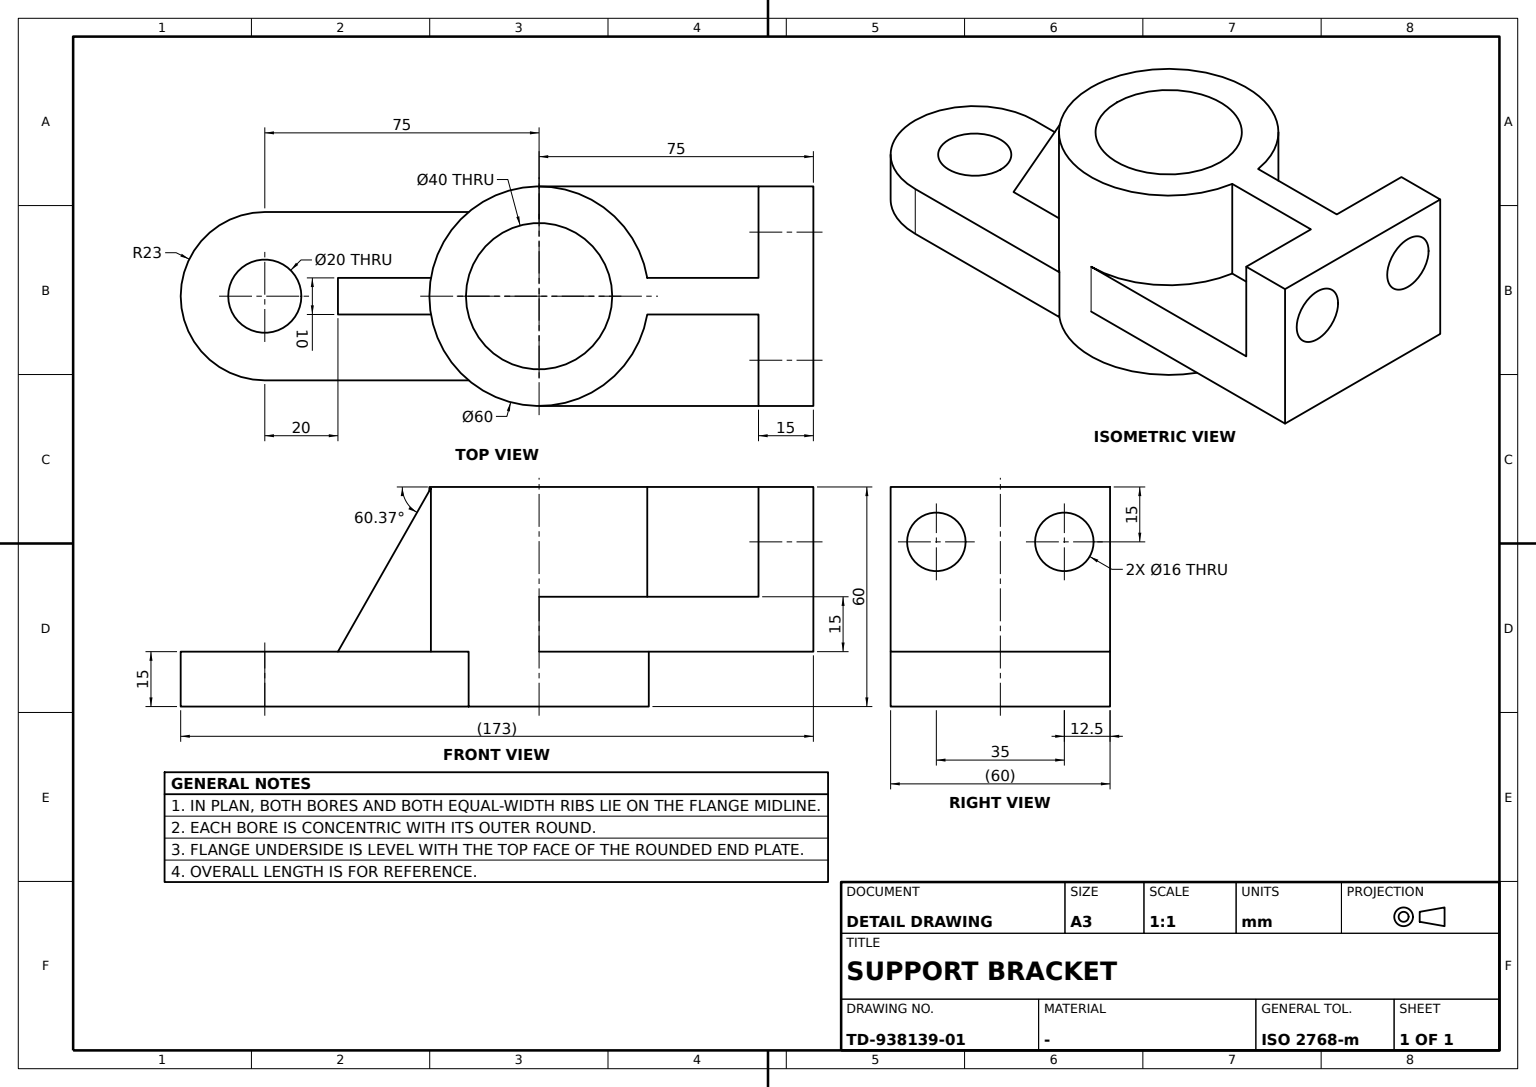
ISO-10303-21;
HEADER;
FILE_DESCRIPTION((''),'2;1');
FILE_NAME('','',(''),(''),'','','');
FILE_SCHEMA(('AUTOMOTIVE_DESIGN'));
ENDSEC;
DATA;
#1=APPLICATION_CONTEXT('');
#2=PRODUCT_CONTEXT('',#1,'mechanical');
#3=PRODUCT('','','',(#2));
#4=PRODUCT_DEFINITION_FORMATION('','',#3);
#5=PRODUCT_DEFINITION_CONTEXT('',#1,'design');
#6=PRODUCT_DEFINITION('','',#4,#5);
#7=PRODUCT_DEFINITION_SHAPE('','',#6);
#8=(LENGTH_UNIT()NAMED_UNIT(*)SI_UNIT(.MILLI.,.METRE.));
#9=(NAMED_UNIT(*)PLANE_ANGLE_UNIT()SI_UNIT($,.RADIAN.));
#10=(NAMED_UNIT(*)SI_UNIT($,.STERADIAN.)SOLID_ANGLE_UNIT());
#11=UNCERTAINTY_MEASURE_WITH_UNIT(LENGTH_MEASURE(1.E-05),#8,'distance_accuracy_value','');
#12=(GEOMETRIC_REPRESENTATION_CONTEXT(3)GLOBAL_UNCERTAINTY_ASSIGNED_CONTEXT((#11))GLOBAL_UNIT_ASSIGNED_CONTEXT((#8,#9,#10))REPRESENTATION_CONTEXT('',''));
#13=CARTESIAN_POINT('',(55.,-5.,15.));
#14=VERTEX_POINT('',#13);
#15=CARTESIAN_POINT('',(55.,5.,15.));
#16=VERTEX_POINT('',#15);
#17=CARTESIAN_POINT('',(55.,0.,15.));
#18=DIRECTION('',(0.,1.,0.));
#19=VECTOR('',#18,1000.);
#20=LINE('',#17,#19);
#21=EDGE_CURVE('',#14,#16,#20,.T.);
#22=ORIENTED_EDGE('',*,*,#21,.T.);
#23=CARTESIAN_POINT('',(29.580399,5.,59.691972));
#24=VERTEX_POINT('',#23);
#25=CARTESIAN_POINT('',(42.290199,5.,37.345986));
#26=DIRECTION('',(0.494398032,0.,-0.869235633));
#27=VECTOR('',#26,1000.);
#28=LINE('',#25,#27);
#29=EDGE_CURVE('',#24,#16,#28,.T.);
#30=ORIENTED_EDGE('',*,*,#29,.F.);
#31=CARTESIAN_POINT('',(30.,0.,58.954242));
#32=VERTEX_POINT('',#31);
#33=CARTESIAN_POINT('',(30.,1.019035,58.954242));
#34=CARTESIAN_POINT('',(29.956732,2.038069,59.030315));
#35=CARTESIAN_POINT('',(29.870188,3.046505,59.182474));
#36=CARTESIAN_POINT('',(29.743385,4.035763,59.405415));
#37=B_SPLINE_CURVE_WITH_KNOTS('',5,(#31,#33,#34,#35,#36,#23),.UNSPECIFIED.,.F.,.F.,(6,6),(0.,7.205662734),.UNSPECIFIED.);
#38=EDGE_CURVE('',#32,#24,#37,.T.);
#39=ORIENTED_EDGE('',*,*,#38,.F.);
#40=CARTESIAN_POINT('',(29.580399,-5.,59.691972));
#41=VERTEX_POINT('',#40);
#42=CARTESIAN_POINT('',(30.,-1.019035,58.954242));
#43=CARTESIAN_POINT('',(29.956732,-2.038069,59.030315));
#44=CARTESIAN_POINT('',(29.870188,-3.046505,59.182474));
#45=CARTESIAN_POINT('',(29.743385,-4.035763,59.405415));
#46=B_SPLINE_CURVE_WITH_KNOTS('',5,(#31,#42,#43,#44,#45,#40),.UNSPECIFIED.,.F.,.F.,(6,6),(0.,7.205662735),.UNSPECIFIED.);
#47=EDGE_CURVE('',#32,#41,#46,.T.);
#48=ORIENTED_EDGE('',*,*,#47,.T.);
#49=CARTESIAN_POINT('',(42.290199,-5.,37.345986));
#50=LINE('',#49,#27);
#51=EDGE_CURVE('',#41,#14,#50,.T.);
#52=ORIENTED_EDGE('',*,*,#51,.T.);
#53=EDGE_LOOP('',(#22,#30,#39,#48,#52));
#54=FACE_OUTER_BOUND('',#53,.T.);
#55=CARTESIAN_POINT('',(29.60858,0.,59.642426));
#56=DIRECTION('',(-0.869235633,0.,-0.494398032));
#57=DIRECTION('',(-0.494398032,0.,0.869235633));
#58=AXIS2_PLACEMENT_3D('',#55,#56,#57);
#59=PLANE('',#58);
#60=ADVANCED_FACE('',(#54),#59,.F.);
#61=CARTESIAN_POINT('',(75.,-23.,0.));
#62=VERTEX_POINT('',#61);
#63=CARTESIAN_POINT('',(19.26136,-23.,0.));
#64=VERTEX_POINT('',#63);
#65=CARTESIAN_POINT('',(47.13068,-23.,0.));
#66=DIRECTION('',(-1.,0.,0.));
#67=VECTOR('',#66,1000.);
#68=LINE('',#65,#67);
#69=EDGE_CURVE('',#62,#64,#68,.T.);
#70=ORIENTED_EDGE('',*,*,#69,.T.);
#71=CARTESIAN_POINT('',(-30.,0.,0.));
#72=VERTEX_POINT('',#71);
#73=CARTESIAN_POINT('',(0.,0.,0.));
#74=DIRECTION('',(0.,0.,1.));
#75=DIRECTION('',(1.,0.,0.));
#76=AXIS2_PLACEMENT_3D('',#73,#74,#75);
#77=CIRCLE('',#76,30.);
#78=EDGE_CURVE('',#72,#64,#77,.T.);
#79=ORIENTED_EDGE('',*,*,#78,.F.);
#80=CARTESIAN_POINT('',(19.26136,23.,0.));
#81=VERTEX_POINT('',#80);
#82=EDGE_CURVE('',#81,#72,#77,.T.);
#83=ORIENTED_EDGE('',*,*,#82,.F.);
#84=CARTESIAN_POINT('',(75.,23.,0.));
#85=VERTEX_POINT('',#84);
#86=CARTESIAN_POINT('',(47.13068,23.,0.));
#87=VECTOR('',#75,1000.);
#88=LINE('',#86,#87);
#89=EDGE_CURVE('',#81,#85,#88,.T.);
#90=ORIENTED_EDGE('',*,*,#89,.T.);
#91=CARTESIAN_POINT('',(98.,0.,0.));
#92=VERTEX_POINT('',#91);
#93=CARTESIAN_POINT('',(75.,0.,0.));
#94=DIRECTION('',(0.,0.,-1.));
#95=AXIS2_PLACEMENT_3D('',#93,#94,#75);
#96=CIRCLE('',#95,23.);
#97=EDGE_CURVE('',#85,#92,#96,.T.);
#98=ORIENTED_EDGE('',*,*,#97,.T.);
#99=EDGE_CURVE('',#92,#62,#96,.T.);
#100=ORIENTED_EDGE('',*,*,#99,.T.);
#101=EDGE_LOOP('',(#70,#79,#83,#90,#98,#100));
#102=FACE_OUTER_BOUND('',#101,.T.);
#103=CARTESIAN_POINT('',(20.,0.,0.));
#104=VERTEX_POINT('',#103);
#105=CARTESIAN_POINT('',(-20.,0.,0.));
#106=VERTEX_POINT('',#105);
#107=CIRCLE('',#76,20.);
#108=EDGE_CURVE('',#104,#106,#107,.T.);
#109=ORIENTED_EDGE('',*,*,#108,.T.);
#110=EDGE_CURVE('',#106,#104,#107,.T.);
#111=ORIENTED_EDGE('',*,*,#110,.T.);
#112=EDGE_LOOP('',(#109,#111));
#113=FACE_BOUND('',#112,.T.);
#114=CARTESIAN_POINT('',(85.,0.,0.));
#115=VERTEX_POINT('',#114);
#116=CARTESIAN_POINT('',(65.,0.,0.));
#117=VERTEX_POINT('',#116);
#118=AXIS2_PLACEMENT_3D('',#93,#74,#75);
#119=CIRCLE('',#118,10.);
#120=EDGE_CURVE('',#115,#117,#119,.T.);
#121=ORIENTED_EDGE('',*,*,#120,.T.);
#122=EDGE_CURVE('',#117,#115,#119,.T.);
#123=ORIENTED_EDGE('',*,*,#122,.T.);
#124=EDGE_LOOP('',(#121,#123));
#125=FACE_BOUND('',#124,.T.);
#126=PLANE('',#76);
#127=ADVANCED_FACE('',(#102,#113,#125),#126,.F.);
#128=CARTESIAN_POINT('',(-75.,-30.,60.));
#129=VERTEX_POINT('',#128);
#130=CARTESIAN_POINT('',(-75.,30.,60.));
#131=VERTEX_POINT('',#130);
#132=CARTESIAN_POINT('',(-75.,0.,60.));
#133=LINE('',#132,#19);
#134=EDGE_CURVE('',#129,#131,#133,.T.);
#135=ORIENTED_EDGE('',*,*,#134,.F.);
#136=CARTESIAN_POINT('',(-60.,-30.,60.));
#137=VERTEX_POINT('',#136);
#138=CARTESIAN_POINT('',(-67.5,-30.,60.));
#139=LINE('',#138,#87);
#140=EDGE_CURVE('',#129,#137,#139,.T.);
#141=ORIENTED_EDGE('',*,*,#140,.T.);
#142=CARTESIAN_POINT('',(-60.,-5.,60.));
#143=VERTEX_POINT('',#142);
#144=CARTESIAN_POINT('',(-60.,-17.5,60.));
#145=LINE('',#144,#19);
#146=EDGE_CURVE('',#137,#143,#145,.T.);
#147=ORIENTED_EDGE('',*,*,#146,.T.);
#148=CARTESIAN_POINT('',(-60.,5.,60.));
#149=VERTEX_POINT('',#148);
#150=CARTESIAN_POINT('',(-60.,0.,60.));
#151=LINE('',#150,#19);
#152=EDGE_CURVE('',#143,#149,#151,.T.);
#153=ORIENTED_EDGE('',*,*,#152,.T.);
#154=CARTESIAN_POINT('',(-60.,30.,60.));
#155=VERTEX_POINT('',#154);
#156=CARTESIAN_POINT('',(-60.,17.5,60.));
#157=LINE('',#156,#19);
#158=EDGE_CURVE('',#149,#155,#157,.T.);
#159=ORIENTED_EDGE('',*,*,#158,.T.);
#160=CARTESIAN_POINT('',(-67.5,30.,60.));
#161=LINE('',#160,#87);
#162=EDGE_CURVE('',#131,#155,#161,.T.);
#163=ORIENTED_EDGE('',*,*,#162,.F.);
#164=EDGE_LOOP('',(#135,#141,#147,#153,#159,#163));
#165=FACE_OUTER_BOUND('',#164,.T.);
#166=CARTESIAN_POINT('',(0.,0.,60.));
#167=AXIS2_PLACEMENT_3D('',#166,#74,#75);
#168=PLANE('',#167);
#169=ADVANCED_FACE('',(#165),#168,.T.);
#170=CARTESIAN_POINT('',(-75.,9.5,45.));
#171=VERTEX_POINT('',#170);
#172=CARTESIAN_POINT('',(-60.,9.5,45.));
#173=VERTEX_POINT('',#172);
#174=CARTESIAN_POINT('',(-67.5,9.5,45.));
#175=LINE('',#174,#87);
#176=EDGE_CURVE('',#171,#173,#175,.T.);
#177=ORIENTED_EDGE('',*,*,#176,.F.);
#178=CARTESIAN_POINT('',(-75.,25.5,45.));
#179=VERTEX_POINT('',#178);
#180=CARTESIAN_POINT('',(-75.,17.5,45.));
#181=DIRECTION('',(0.,-1.,0.));
#182=AXIS2_PLACEMENT_3D('',#180,#66,#181);
#183=CIRCLE('',#182,8.);
#184=EDGE_CURVE('',#171,#179,#183,.T.);
#185=ORIENTED_EDGE('',*,*,#184,.T.);
#186=CARTESIAN_POINT('',(-60.,25.5,45.));
#187=VERTEX_POINT('',#186);
#188=CARTESIAN_POINT('',(-67.5,25.5,45.));
#189=LINE('',#188,#87);
#190=EDGE_CURVE('',#179,#187,#189,.T.);
#191=ORIENTED_EDGE('',*,*,#190,.T.);
#192=CARTESIAN_POINT('',(-60.,17.5,45.));
#193=AXIS2_PLACEMENT_3D('',#192,#66,#181);
#194=CIRCLE('',#193,8.);
#195=EDGE_CURVE('',#173,#187,#194,.T.);
#196=ORIENTED_EDGE('',*,*,#195,.F.);
#197=EDGE_LOOP('',(#177,#185,#191,#196));
#198=FACE_OUTER_BOUND('',#197,.T.);
#199=CARTESIAN_POINT('',(-67.5,17.5,45.));
#200=AXIS2_PLACEMENT_3D('',#199,#75,#181);
#201=CYLINDRICAL_SURFACE('',#200,8.);
#202=ADVANCED_FACE('',(#198),#201,.F.);
#203=CARTESIAN_POINT('',(-60.,-5.,30.));
#204=VERTEX_POINT('',#203);
#205=CARTESIAN_POINT('',(-29.580399,-5.,30.));
#206=VERTEX_POINT('',#205);
#207=CARTESIAN_POINT('',(-44.790199,-5.,30.));
#208=LINE('',#207,#87);
#209=EDGE_CURVE('',#204,#206,#208,.T.);
#210=ORIENTED_EDGE('',*,*,#209,.T.);
#211=CARTESIAN_POINT('',(-29.580399,-5.,60.));
#212=VERTEX_POINT('',#211);
#213=CARTESIAN_POINT('',(-29.580399,-5.,45.));
#214=VECTOR('',#74,1000.);
#215=LINE('',#213,#214);
#216=EDGE_CURVE('',#206,#212,#215,.T.);
#217=ORIENTED_EDGE('',*,*,#216,.T.);
#218=CARTESIAN_POINT('',(-29.795248,-5.,60.));
#219=VERTEX_POINT('',#218);
#220=CARTESIAN_POINT('',(-29.687823,-5.,60.));
#221=LINE('',#220,#67);
#222=EDGE_CURVE('',#212,#219,#221,.T.);
#223=ORIENTED_EDGE('',*,*,#222,.T.);
#224=CARTESIAN_POINT('',(-44.897624,-5.,60.));
#225=LINE('',#224,#67);
#226=EDGE_CURVE('',#219,#143,#225,.T.);
#227=ORIENTED_EDGE('',*,*,#226,.T.);
#228=CARTESIAN_POINT('',(-60.,-5.,45.));
#229=VECTOR('',#94,1000.);
#230=LINE('',#228,#229);
#231=EDGE_CURVE('',#143,#204,#230,.T.);
#232=ORIENTED_EDGE('',*,*,#231,.T.);
#233=EDGE_LOOP('',(#210,#217,#223,#227,#232));
#234=FACE_OUTER_BOUND('',#233,.T.);
#235=CARTESIAN_POINT('',(0.,-5.,0.));
#236=AXIS2_PLACEMENT_3D('',#235,#18,#66);
#237=PLANE('',#236);
#238=ADVANCED_FACE('',(#234),#237,.F.);
#239=ORIENTED_EDGE('',*,*,#78,.T.);
#240=CARTESIAN_POINT('',(19.26136,-23.,15.));
#241=VERTEX_POINT('',#240);
#242=CARTESIAN_POINT('',(19.26136,-23.,7.5));
#243=LINE('',#242,#229);
#244=EDGE_CURVE('',#241,#64,#243,.T.);
#245=ORIENTED_EDGE('',*,*,#244,.F.);
#246=CARTESIAN_POINT('',(29.580399,-5.,15.));
#247=VERTEX_POINT('',#246);
#248=CARTESIAN_POINT('',(0.,0.,15.));
#249=AXIS2_PLACEMENT_3D('',#248,#94,#75);
#250=CIRCLE('',#249,30.);
#251=EDGE_CURVE('',#247,#241,#250,.T.);
#252=ORIENTED_EDGE('',*,*,#251,.F.);
#253=CARTESIAN_POINT('',(29.580399,-5.,37.345986));
#254=LINE('',#253,#214);
#255=EDGE_CURVE('',#247,#41,#254,.T.);
#256=ORIENTED_EDGE('',*,*,#255,.T.);
#257=ORIENTED_EDGE('',*,*,#47,.F.);
#258=CARTESIAN_POINT('',(30.,0.,60.));
#259=VERTEX_POINT('',#258);
#260=CARTESIAN_POINT('',(30.,0.,30.));
#261=LINE('',#260,#214);
#262=EDGE_CURVE('',#32,#259,#261,.T.);
#263=ORIENTED_EDGE('',*,*,#262,.T.);
#264=CIRCLE('',#167,30.);
#265=EDGE_CURVE('',#212,#259,#264,.T.);
#266=ORIENTED_EDGE('',*,*,#265,.F.);
#267=ORIENTED_EDGE('',*,*,#216,.F.);
#268=CARTESIAN_POINT('',(0.,-30.,30.));
#269=VERTEX_POINT('',#268);
#270=CARTESIAN_POINT('',(0.,0.,30.));
#271=AXIS2_PLACEMENT_3D('',#270,#74,#75);
#272=CIRCLE('',#271,30.);
#273=EDGE_CURVE('',#206,#269,#272,.T.);
#274=ORIENTED_EDGE('',*,*,#273,.T.);
#275=CARTESIAN_POINT('',(0.,-30.,15.));
#276=VERTEX_POINT('',#275);
#277=CARTESIAN_POINT('',(0.,-30.,22.5));
#278=LINE('',#277,#214);
#279=EDGE_CURVE('',#276,#269,#278,.T.);
#280=ORIENTED_EDGE('',*,*,#279,.F.);
#281=CARTESIAN_POINT('',(-30.,0.,15.));
#282=VERTEX_POINT('',#281);
#283=AXIS2_PLACEMENT_3D('',#248,#74,#75);
#284=CIRCLE('',#283,30.);
#285=EDGE_CURVE('',#282,#276,#284,.T.);
#286=ORIENTED_EDGE('',*,*,#285,.F.);
#287=CARTESIAN_POINT('',(-30.,0.,30.));
#288=LINE('',#287,#214);
#289=EDGE_CURVE('',#72,#282,#288,.T.);
#290=ORIENTED_EDGE('',*,*,#289,.F.);
#291=EDGE_LOOP('',(#239,#245,#252,#256,#257,#263,#266,#267,#274,#280,#286,#290));
#292=FACE_OUTER_BOUND('',#291,.T.);
#293=AXIS2_PLACEMENT_3D('',#270,#94,#75);
#294=CYLINDRICAL_SURFACE('',#293,30.);
#295=ADVANCED_FACE('',(#292),#294,.T.);
#296=CARTESIAN_POINT('',(-29.580399,5.,30.));
#297=VERTEX_POINT('',#296);
#298=CARTESIAN_POINT('',(-29.580399,5.,60.));
#299=VERTEX_POINT('',#298);
#300=CARTESIAN_POINT('',(-29.580399,5.,45.));
#301=LINE('',#300,#214);
#302=EDGE_CURVE('',#297,#299,#301,.T.);
#303=ORIENTED_EDGE('',*,*,#302,.F.);
#304=CARTESIAN_POINT('',(-60.,5.,30.));
#305=VERTEX_POINT('',#304);
#306=CARTESIAN_POINT('',(-44.790199,5.,30.));
#307=LINE('',#306,#87);
#308=EDGE_CURVE('',#305,#297,#307,.T.);
#309=ORIENTED_EDGE('',*,*,#308,.F.);
#310=CARTESIAN_POINT('',(-60.,5.,45.));
#311=LINE('',#310,#229);
#312=EDGE_CURVE('',#149,#305,#311,.T.);
#313=ORIENTED_EDGE('',*,*,#312,.F.);
#314=CARTESIAN_POINT('',(-29.795248,5.,60.));
#315=VERTEX_POINT('',#314);
#316=CARTESIAN_POINT('',(-44.897624,5.,60.));
#317=LINE('',#316,#67);
#318=EDGE_CURVE('',#315,#149,#317,.T.);
#319=ORIENTED_EDGE('',*,*,#318,.F.);
#320=CARTESIAN_POINT('',(-29.687823,5.,60.));
#321=LINE('',#320,#67);
#322=EDGE_CURVE('',#299,#315,#321,.T.);
#323=ORIENTED_EDGE('',*,*,#322,.F.);
#324=EDGE_LOOP('',(#303,#309,#313,#319,#323));
#325=FACE_OUTER_BOUND('',#324,.T.);
#326=CARTESIAN_POINT('',(0.,5.,0.));
#327=AXIS2_PLACEMENT_3D('',#326,#18,#66);
#328=PLANE('',#327);
#329=ADVANCED_FACE('',(#325),#328,.T.);
#330=CARTESIAN_POINT('',(19.26136,23.,15.));
#331=VERTEX_POINT('',#330);
#332=CARTESIAN_POINT('',(75.,23.,15.));
#333=VERTEX_POINT('',#332);
#334=CARTESIAN_POINT('',(47.13068,23.,15.));
#335=LINE('',#334,#87);
#336=EDGE_CURVE('',#331,#333,#335,.T.);
#337=ORIENTED_EDGE('',*,*,#336,.T.);
#338=CARTESIAN_POINT('',(75.,23.,7.5));
#339=LINE('',#338,#214);
#340=EDGE_CURVE('',#85,#333,#339,.T.);
#341=ORIENTED_EDGE('',*,*,#340,.F.);
#342=ORIENTED_EDGE('',*,*,#89,.F.);
#343=CARTESIAN_POINT('',(19.26136,23.,7.5));
#344=LINE('',#343,#229);
#345=EDGE_CURVE('',#331,#81,#344,.T.);
#346=ORIENTED_EDGE('',*,*,#345,.F.);
#347=EDGE_LOOP('',(#337,#341,#342,#346));
#348=FACE_OUTER_BOUND('',#347,.T.);
#349=AXIS2_PLACEMENT_3D('',#80,#181,#75);
#350=PLANE('',#349);
#351=ADVANCED_FACE('',(#348),#350,.F.);
#352=ORIENTED_EDGE('',*,*,#29,.T.);
#353=CARTESIAN_POINT('',(29.580399,5.,15.));
#354=VERTEX_POINT('',#353);
#355=CARTESIAN_POINT('',(42.290199,5.,15.));
#356=LINE('',#355,#87);
#357=EDGE_CURVE('',#354,#16,#356,.T.);
#358=ORIENTED_EDGE('',*,*,#357,.F.);
#359=CARTESIAN_POINT('',(29.580399,5.,37.345986));
#360=LINE('',#359,#214);
#361=EDGE_CURVE('',#354,#24,#360,.T.);
#362=ORIENTED_EDGE('',*,*,#361,.T.);
#363=EDGE_LOOP('',(#352,#358,#362));
#364=FACE_OUTER_BOUND('',#363,.T.);
#365=ADVANCED_FACE('',(#364),#328,.T.);
#366=CARTESIAN_POINT('',(-60.,-9.5,45.));
#367=VERTEX_POINT('',#366);
#368=CARTESIAN_POINT('',(-60.,-25.5,45.));
#369=VERTEX_POINT('',#368);
#370=CARTESIAN_POINT('',(-60.,-17.5,45.));
#371=AXIS2_PLACEMENT_3D('',#370,#66,#181);
#372=CIRCLE('',#371,8.);
#373=EDGE_CURVE('',#367,#369,#372,.T.);
#374=ORIENTED_EDGE('',*,*,#373,.T.);
#375=EDGE_CURVE('',#369,#367,#372,.T.);
#376=ORIENTED_EDGE('',*,*,#375,.T.);
#377=EDGE_LOOP('',(#374,#376));
#378=FACE_BOUND('',#377,.T.);
#379=ORIENTED_EDGE('',*,*,#231,.F.);
#380=ORIENTED_EDGE('',*,*,#146,.F.);
#381=CARTESIAN_POINT('',(-60.,-30.,30.));
#382=VERTEX_POINT('',#381);
#383=CARTESIAN_POINT('',(-60.,-30.,45.));
#384=LINE('',#383,#214);
#385=EDGE_CURVE('',#382,#137,#384,.T.);
#386=ORIENTED_EDGE('',*,*,#385,.F.);
#387=CARTESIAN_POINT('',(-60.,-17.5,30.));
#388=VECTOR('',#181,1000.);
#389=LINE('',#387,#388);
#390=EDGE_CURVE('',#204,#382,#389,.T.);
#391=ORIENTED_EDGE('',*,*,#390,.F.);
#392=EDGE_LOOP('',(#379,#380,#386,#391));
#393=FACE_OUTER_BOUND('',#392,.T.);
#394=CARTESIAN_POINT('',(-60.,0.,0.));
#395=AXIS2_PLACEMENT_3D('',#394,#66,#181);
#396=PLANE('',#395);
#397=ADVANCED_FACE('',(#378,#393),#396,.F.);
#398=ORIENTED_EDGE('',*,*,#308,.T.);
#399=CARTESIAN_POINT('',(0.,30.,30.));
#400=VERTEX_POINT('',#399);
#401=EDGE_CURVE('',#400,#297,#272,.T.);
#402=ORIENTED_EDGE('',*,*,#401,.F.);
#403=CARTESIAN_POINT('',(-60.,30.,30.));
#404=VERTEX_POINT('',#403);
#405=CARTESIAN_POINT('',(-30.,30.,30.));
#406=LINE('',#405,#87);
#407=EDGE_CURVE('',#404,#400,#406,.T.);
#408=ORIENTED_EDGE('',*,*,#407,.F.);
#409=CARTESIAN_POINT('',(-60.,17.5,30.));
#410=LINE('',#409,#388);
#411=EDGE_CURVE('',#404,#305,#410,.T.);
#412=ORIENTED_EDGE('',*,*,#411,.T.);
#413=EDGE_LOOP('',(#398,#402,#408,#412));
#414=FACE_OUTER_BOUND('',#413,.T.);
#415=PLANE('',#293);
#416=ADVANCED_FACE('',(#414),#415,.F.);
#417=ORIENTED_EDGE('',*,*,#411,.F.);
#418=CARTESIAN_POINT('',(-60.,30.,45.));
#419=LINE('',#418,#229);
#420=EDGE_CURVE('',#155,#404,#419,.T.);
#421=ORIENTED_EDGE('',*,*,#420,.F.);
#422=ORIENTED_EDGE('',*,*,#158,.F.);
#423=ORIENTED_EDGE('',*,*,#312,.T.);
#424=EDGE_LOOP('',(#417,#421,#422,#423));
#425=FACE_OUTER_BOUND('',#424,.T.);
#426=ORIENTED_EDGE('',*,*,#195,.T.);
#427=EDGE_CURVE('',#187,#173,#194,.T.);
#428=ORIENTED_EDGE('',*,*,#427,.T.);
#429=EDGE_LOOP('',(#426,#428));
#430=FACE_BOUND('',#429,.T.);
#431=ADVANCED_FACE('',(#425,#430),#396,.F.);
#432=CARTESIAN_POINT('',(85.,0.,15.));
#433=VERTEX_POINT('',#432);
#434=CARTESIAN_POINT('',(85.,0.,7.5));
#435=LINE('',#434,#229);
#436=EDGE_CURVE('',#433,#115,#435,.T.);
#437=ORIENTED_EDGE('',*,*,#436,.T.);
#438=ORIENTED_EDGE('',*,*,#122,.F.);
#439=CARTESIAN_POINT('',(65.,0.,15.));
#440=VERTEX_POINT('',#439);
#441=CARTESIAN_POINT('',(65.,0.,7.5));
#442=LINE('',#441,#229);
#443=EDGE_CURVE('',#440,#117,#442,.T.);
#444=ORIENTED_EDGE('',*,*,#443,.F.);
#445=CARTESIAN_POINT('',(75.,0.,15.));
#446=AXIS2_PLACEMENT_3D('',#445,#74,#75);
#447=CIRCLE('',#446,10.);
#448=EDGE_CURVE('',#440,#433,#447,.T.);
#449=ORIENTED_EDGE('',*,*,#448,.T.);
#450=EDGE_LOOP('',(#437,#438,#444,#449));
#451=FACE_OUTER_BOUND('',#450,.T.);
#452=CARTESIAN_POINT('',(75.,0.,7.5));
#453=AXIS2_PLACEMENT_3D('',#452,#94,#75);
#454=CYLINDRICAL_SURFACE('',#453,10.);
#455=ADVANCED_FACE('',(#451),#454,.F.);
#456=ORIENTED_EDGE('',*,*,#273,.F.);
#457=ORIENTED_EDGE('',*,*,#209,.F.);
#458=ORIENTED_EDGE('',*,*,#390,.T.);
#459=CARTESIAN_POINT('',(-30.,-30.,30.));
#460=LINE('',#459,#67);
#461=EDGE_CURVE('',#269,#382,#460,.T.);
#462=ORIENTED_EDGE('',*,*,#461,.F.);
#463=EDGE_LOOP('',(#456,#457,#458,#462));
#464=FACE_OUTER_BOUND('',#463,.T.);
#465=ADVANCED_FACE('',(#464),#415,.F.);
#466=CARTESIAN_POINT('',(-75.,-30.,15.));
#467=VERTEX_POINT('',#466);
#468=CARTESIAN_POINT('',(-75.,30.,15.));
#469=VERTEX_POINT('',#468);
#470=CARTESIAN_POINT('',(-75.,0.,15.));
#471=LINE('',#470,#19);
#472=EDGE_CURVE('',#467,#469,#471,.T.);
#473=ORIENTED_EDGE('',*,*,#472,.T.);
#474=CARTESIAN_POINT('',(0.,30.,15.));
#475=VERTEX_POINT('',#474);
#476=CARTESIAN_POINT('',(-37.5,30.,15.));
#477=LINE('',#476,#87);
#478=EDGE_CURVE('',#469,#475,#477,.T.);
#479=ORIENTED_EDGE('',*,*,#478,.T.);
#480=EDGE_CURVE('',#475,#282,#284,.T.);
#481=ORIENTED_EDGE('',*,*,#480,.T.);
#482=ORIENTED_EDGE('',*,*,#285,.T.);
#483=CARTESIAN_POINT('',(-37.5,-30.,15.));
#484=LINE('',#483,#67);
#485=EDGE_CURVE('',#276,#467,#484,.T.);
#486=ORIENTED_EDGE('',*,*,#485,.T.);
#487=EDGE_LOOP('',(#473,#479,#481,#482,#486));
#488=FACE_OUTER_BOUND('',#487,.T.);
#489=PLANE('',#249);
#490=ADVANCED_FACE('',(#488),#489,.T.);
#491=CARTESIAN_POINT('',(-75.,-30.,37.5));
#492=LINE('',#491,#214);
#493=EDGE_CURVE('',#467,#129,#492,.T.);
#494=ORIENTED_EDGE('',*,*,#493,.T.);
#495=ORIENTED_EDGE('',*,*,#134,.T.);
#496=CARTESIAN_POINT('',(-75.,30.,37.5));
#497=LINE('',#496,#214);
#498=EDGE_CURVE('',#469,#131,#497,.T.);
#499=ORIENTED_EDGE('',*,*,#498,.F.);
#500=ORIENTED_EDGE('',*,*,#472,.F.);
#501=EDGE_LOOP('',(#494,#495,#499,#500));
#502=FACE_OUTER_BOUND('',#501,.T.);
#503=CARTESIAN_POINT('',(-75.,-25.5,45.));
#504=VERTEX_POINT('',#503);
#505=CARTESIAN_POINT('',(-75.,-9.5,45.));
#506=VERTEX_POINT('',#505);
#507=CARTESIAN_POINT('',(-75.,-17.5,45.));
#508=AXIS2_PLACEMENT_3D('',#507,#66,#181);
#509=CIRCLE('',#508,8.);
#510=EDGE_CURVE('',#504,#506,#509,.T.);
#511=ORIENTED_EDGE('',*,*,#510,.F.);
#512=EDGE_CURVE('',#506,#504,#509,.T.);
#513=ORIENTED_EDGE('',*,*,#512,.F.);
#514=EDGE_LOOP('',(#511,#513));
#515=FACE_BOUND('',#514,.T.);
#516=ORIENTED_EDGE('',*,*,#184,.F.);
#517=EDGE_CURVE('',#179,#171,#183,.T.);
#518=ORIENTED_EDGE('',*,*,#517,.F.);
#519=EDGE_LOOP('',(#516,#518));
#520=FACE_BOUND('',#519,.T.);
#521=AXIS2_PLACEMENT_3D('',#466,#75,#18);
#522=PLANE('',#521);
#523=ADVANCED_FACE('',(#502,#515,#520),#522,.F.);
#524=CARTESIAN_POINT('',(20.,0.,60.));
#525=VERTEX_POINT('',#524);
#526=CARTESIAN_POINT('',(-20.,0.,60.));
#527=VERTEX_POINT('',#526);
#528=CIRCLE('',#167,20.);
#529=EDGE_CURVE('',#525,#527,#528,.T.);
#530=ORIENTED_EDGE('',*,*,#529,.F.);
#531=EDGE_CURVE('',#527,#525,#528,.T.);
#532=ORIENTED_EDGE('',*,*,#531,.F.);
#533=EDGE_LOOP('',(#530,#532));
#534=FACE_BOUND('',#533,.T.);
#535=ORIENTED_EDGE('',*,*,#265,.T.);
#536=EDGE_CURVE('',#259,#299,#264,.T.);
#537=ORIENTED_EDGE('',*,*,#536,.T.);
#538=ORIENTED_EDGE('',*,*,#322,.T.);
#539=CARTESIAN_POINT('',(-29.795248,0.,60.));
#540=LINE('',#539,#19);
#541=EDGE_CURVE('',#219,#315,#540,.T.);
#542=ORIENTED_EDGE('',*,*,#541,.F.);
#543=ORIENTED_EDGE('',*,*,#222,.F.);
#544=EDGE_LOOP('',(#535,#537,#538,#542,#543));
#545=FACE_OUTER_BOUND('',#544,.T.);
#546=ADVANCED_FACE('',(#534,#545),#168,.T.);
#547=ORIENTED_EDGE('',*,*,#110,.F.);
#548=CARTESIAN_POINT('',(-20.,0.,30.));
#549=LINE('',#548,#229);
#550=EDGE_CURVE('',#527,#106,#549,.T.);
#551=ORIENTED_EDGE('',*,*,#550,.F.);
#552=ORIENTED_EDGE('',*,*,#531,.T.);
#553=CARTESIAN_POINT('',(20.,0.,30.));
#554=LINE('',#553,#229);
#555=EDGE_CURVE('',#525,#104,#554,.T.);
#556=ORIENTED_EDGE('',*,*,#555,.T.);
#557=EDGE_LOOP('',(#547,#551,#552,#556));
#558=FACE_OUTER_BOUND('',#557,.T.);
#559=CYLINDRICAL_SURFACE('',#293,20.);
#560=ADVANCED_FACE('',(#558),#559,.F.);
#561=ORIENTED_EDGE('',*,*,#69,.F.);
#562=CARTESIAN_POINT('',(75.,-23.,15.));
#563=VERTEX_POINT('',#562);
#564=CARTESIAN_POINT('',(75.,-23.,7.5));
#565=LINE('',#564,#214);
#566=EDGE_CURVE('',#62,#563,#565,.T.);
#567=ORIENTED_EDGE('',*,*,#566,.T.);
#568=CARTESIAN_POINT('',(47.13068,-23.,15.));
#569=LINE('',#568,#67);
#570=EDGE_CURVE('',#563,#241,#569,.T.);
#571=ORIENTED_EDGE('',*,*,#570,.T.);
#572=ORIENTED_EDGE('',*,*,#244,.T.);
#573=EDGE_LOOP('',(#561,#567,#571,#572));
#574=FACE_OUTER_BOUND('',#573,.T.);
#575=AXIS2_PLACEMENT_3D('',#63,#181,#75);
#576=PLANE('',#575);
#577=ADVANCED_FACE('',(#574),#576,.T.);
#578=CARTESIAN_POINT('',(42.290199,-5.,15.));
#579=LINE('',#578,#87);
#580=EDGE_CURVE('',#247,#14,#579,.T.);
#581=ORIENTED_EDGE('',*,*,#580,.T.);
#582=ORIENTED_EDGE('',*,*,#51,.F.);
#583=ORIENTED_EDGE('',*,*,#255,.F.);
#584=EDGE_LOOP('',(#581,#582,#583));
#585=FACE_OUTER_BOUND('',#584,.T.);
#586=ADVANCED_FACE('',(#585),#237,.F.);
#587=ORIENTED_EDGE('',*,*,#485,.F.);
#588=ORIENTED_EDGE('',*,*,#279,.T.);
#589=ORIENTED_EDGE('',*,*,#461,.T.);
#590=ORIENTED_EDGE('',*,*,#385,.T.);
#591=ORIENTED_EDGE('',*,*,#140,.F.);
#592=ORIENTED_EDGE('',*,*,#493,.F.);
#593=EDGE_LOOP('',(#587,#588,#589,#590,#591,#592));
#594=FACE_OUTER_BOUND('',#593,.T.);
#595=AXIS2_PLACEMENT_3D('',#275,#18,#66);
#596=PLANE('',#595);
#597=ADVANCED_FACE('',(#594),#596,.F.);
#598=ORIENTED_EDGE('',*,*,#226,.F.);
#599=ORIENTED_EDGE('',*,*,#541,.T.);
#600=ORIENTED_EDGE('',*,*,#318,.T.);
#601=ORIENTED_EDGE('',*,*,#152,.F.);
#602=EDGE_LOOP('',(#598,#599,#600,#601));
#603=FACE_OUTER_BOUND('',#602,.T.);
#604=ADVANCED_FACE('',(#603),#168,.T.);
#605=ORIENTED_EDGE('',*,*,#99,.F.);
#606=CARTESIAN_POINT('',(98.,0.,15.));
#607=VERTEX_POINT('',#606);
#608=CARTESIAN_POINT('',(98.,0.,7.5));
#609=LINE('',#608,#214);
#610=EDGE_CURVE('',#92,#607,#609,.T.);
#611=ORIENTED_EDGE('',*,*,#610,.T.);
#612=AXIS2_PLACEMENT_3D('',#445,#94,#75);
#613=CIRCLE('',#612,23.);
#614=EDGE_CURVE('',#607,#563,#613,.T.);
#615=ORIENTED_EDGE('',*,*,#614,.T.);
#616=ORIENTED_EDGE('',*,*,#566,.F.);
#617=EDGE_LOOP('',(#605,#611,#615,#616));
#618=FACE_OUTER_BOUND('',#617,.T.);
#619=AXIS2_PLACEMENT_3D('',#452,#74,#75);
#620=CYLINDRICAL_SURFACE('',#619,23.);
#621=ADVANCED_FACE('',(#618),#620,.T.);
#622=EDGE_CURVE('',#433,#440,#447,.T.);
#623=ORIENTED_EDGE('',*,*,#622,.F.);
#624=ORIENTED_EDGE('',*,*,#448,.F.);
#625=EDGE_LOOP('',(#623,#624));
#626=FACE_BOUND('',#625,.T.);
#627=ORIENTED_EDGE('',*,*,#21,.F.);
#628=ORIENTED_EDGE('',*,*,#580,.F.);
#629=ORIENTED_EDGE('',*,*,#251,.T.);
#630=ORIENTED_EDGE('',*,*,#570,.F.);
#631=ORIENTED_EDGE('',*,*,#614,.F.);
#632=EDGE_CURVE('',#333,#607,#613,.T.);
#633=ORIENTED_EDGE('',*,*,#632,.F.);
#634=ORIENTED_EDGE('',*,*,#336,.F.);
#635=EDGE_CURVE('',#331,#354,#250,.T.);
#636=ORIENTED_EDGE('',*,*,#635,.T.);
#637=ORIENTED_EDGE('',*,*,#357,.T.);
#638=EDGE_LOOP('',(#627,#628,#629,#630,#631,#633,#634,#636,#637));
#639=FACE_OUTER_BOUND('',#638,.T.);
#640=ADVANCED_FACE('',(#626,#639),#489,.F.);
#641=ORIENTED_EDGE('',*,*,#262,.F.);
#642=ORIENTED_EDGE('',*,*,#38,.T.);
#643=ORIENTED_EDGE('',*,*,#361,.F.);
#644=ORIENTED_EDGE('',*,*,#635,.F.);
#645=ORIENTED_EDGE('',*,*,#345,.T.);
#646=ORIENTED_EDGE('',*,*,#82,.T.);
#647=ORIENTED_EDGE('',*,*,#289,.T.);
#648=ORIENTED_EDGE('',*,*,#480,.F.);
#649=CARTESIAN_POINT('',(0.,30.,22.5));
#650=LINE('',#649,#214);
#651=EDGE_CURVE('',#475,#400,#650,.T.);
#652=ORIENTED_EDGE('',*,*,#651,.T.);
#653=ORIENTED_EDGE('',*,*,#401,.T.);
#654=ORIENTED_EDGE('',*,*,#302,.T.);
#655=ORIENTED_EDGE('',*,*,#536,.F.);
#656=EDGE_LOOP('',(#641,#642,#643,#644,#645,#646,#647,#648,#652,#653,#654,#655));
#657=FACE_OUTER_BOUND('',#656,.T.);
#658=ADVANCED_FACE('',(#657),#294,.T.);
#659=ORIENTED_EDGE('',*,*,#420,.T.);
#660=ORIENTED_EDGE('',*,*,#407,.T.);
#661=ORIENTED_EDGE('',*,*,#651,.F.);
#662=ORIENTED_EDGE('',*,*,#478,.F.);
#663=ORIENTED_EDGE('',*,*,#498,.T.);
#664=ORIENTED_EDGE('',*,*,#162,.T.);
#665=EDGE_LOOP('',(#659,#660,#661,#662,#663,#664));
#666=FACE_OUTER_BOUND('',#665,.T.);
#667=AXIS2_PLACEMENT_3D('',#474,#18,#66);
#668=PLANE('',#667);
#669=ADVANCED_FACE('',(#666),#668,.T.);
#670=ORIENTED_EDGE('',*,*,#190,.F.);
#671=ORIENTED_EDGE('',*,*,#517,.T.);
#672=ORIENTED_EDGE('',*,*,#176,.T.);
#673=ORIENTED_EDGE('',*,*,#427,.F.);
#674=EDGE_LOOP('',(#670,#671,#672,#673));
#675=FACE_OUTER_BOUND('',#674,.T.);
#676=ADVANCED_FACE('',(#675),#201,.F.);
#677=CARTESIAN_POINT('',(-67.5,-9.5,45.));
#678=LINE('',#677,#87);
#679=EDGE_CURVE('',#506,#367,#678,.T.);
#680=ORIENTED_EDGE('',*,*,#679,.T.);
#681=ORIENTED_EDGE('',*,*,#375,.F.);
#682=CARTESIAN_POINT('',(-67.5,-25.5,45.));
#683=LINE('',#682,#87);
#684=EDGE_CURVE('',#504,#369,#683,.T.);
#685=ORIENTED_EDGE('',*,*,#684,.F.);
#686=ORIENTED_EDGE('',*,*,#510,.T.);
#687=EDGE_LOOP('',(#680,#681,#685,#686));
#688=FACE_OUTER_BOUND('',#687,.T.);
#689=CARTESIAN_POINT('',(-67.5,-17.5,45.));
#690=AXIS2_PLACEMENT_3D('',#689,#75,#181);
#691=CYLINDRICAL_SURFACE('',#690,8.);
#692=ADVANCED_FACE('',(#688),#691,.F.);
#693=ORIENTED_EDGE('',*,*,#679,.F.);
#694=ORIENTED_EDGE('',*,*,#512,.T.);
#695=ORIENTED_EDGE('',*,*,#684,.T.);
#696=ORIENTED_EDGE('',*,*,#373,.F.);
#697=EDGE_LOOP('',(#693,#694,#695,#696));
#698=FACE_OUTER_BOUND('',#697,.T.);
#699=ADVANCED_FACE('',(#698),#691,.F.);
#700=ORIENTED_EDGE('',*,*,#622,.T.);
#701=ORIENTED_EDGE('',*,*,#443,.T.);
#702=ORIENTED_EDGE('',*,*,#120,.F.);
#703=ORIENTED_EDGE('',*,*,#436,.F.);
#704=EDGE_LOOP('',(#700,#701,#702,#703));
#705=FACE_OUTER_BOUND('',#704,.T.);
#706=ADVANCED_FACE('',(#705),#454,.F.);
#707=ORIENTED_EDGE('',*,*,#529,.T.);
#708=ORIENTED_EDGE('',*,*,#550,.T.);
#709=ORIENTED_EDGE('',*,*,#108,.F.);
#710=ORIENTED_EDGE('',*,*,#555,.F.);
#711=EDGE_LOOP('',(#707,#708,#709,#710));
#712=FACE_OUTER_BOUND('',#711,.T.);
#713=ADVANCED_FACE('',(#712),#559,.F.);
#714=ORIENTED_EDGE('',*,*,#340,.T.);
#715=ORIENTED_EDGE('',*,*,#632,.T.);
#716=ORIENTED_EDGE('',*,*,#610,.F.);
#717=ORIENTED_EDGE('',*,*,#97,.F.);
#718=EDGE_LOOP('',(#714,#715,#716,#717));
#719=FACE_OUTER_BOUND('',#718,.T.);
#720=ADVANCED_FACE('',(#719),#620,.T.);
#721=CLOSED_SHELL('',(#60,#127,#169,#202,#238,#295,#329,#351,#365,#397,#416,#431,#455,#465,#490,#523,#546,#560,#577,#586,#597,#604,#621,#640,#658,#669,#676,#692,#699,#706,#713,#720));
#722=MANIFOLD_SOLID_BREP('',#721);
#723=ADVANCED_BREP_SHAPE_REPRESENTATION('',(#722),#12);
#724=SHAPE_DEFINITION_REPRESENTATION(#7,#723);
ENDSEC;
END-ISO-10303-21;
